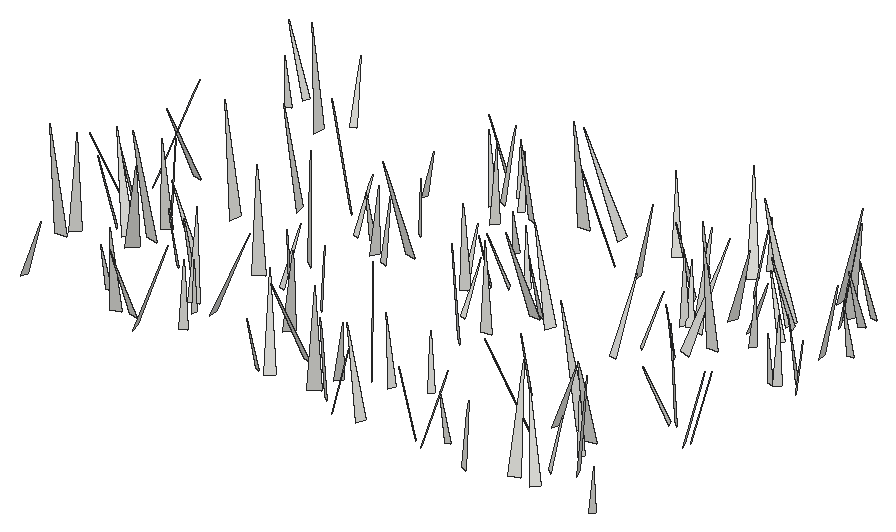
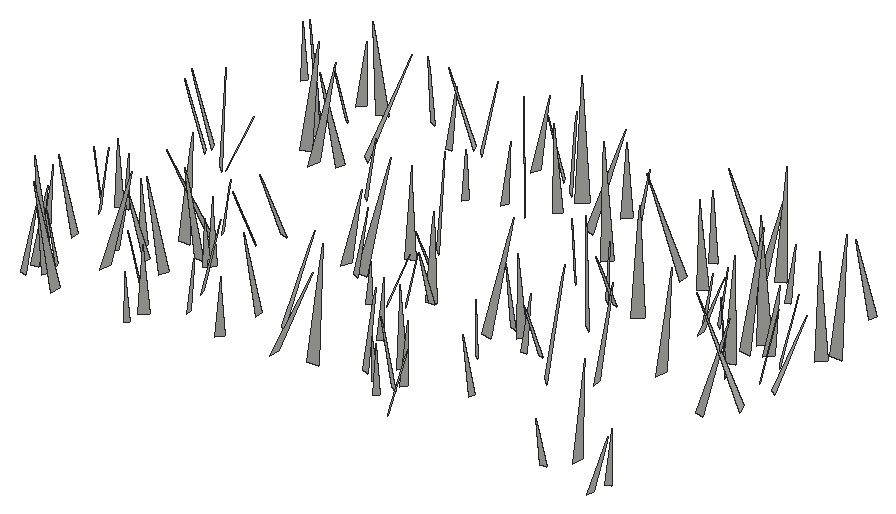
# SketchUp Ruby script. Lengths in inches.
U = 1.inch
M = Sketchup.active_model
def pt(a) = Geom::Point3d.new(a.map { |v| v * U })
def face(e, loops, mat)
  f = e.add_face(loops[0].map { |a| pt(a) })
  loops[1..].each { |l| e.add_face(l.map { |a| pt(a) }).erase! }
  f.material = f.back_material = mat if mat
  f
end
# faces: each face lists its corners as indices into pts; further lists are holes
def faces(e, pts, list, mat = nil) = list.each { |f| face(e, (f[0].is_a?(Array) ? f : [f]).map { |l| l.map { |i| pts[i] } }, mat) }
# xy, xz, yz: faces in a plane at the given z, y or x. An outline is a flat list of corners, or four numbers for a rectangle; further outlines are holes
def ring(l) = l.size == 4 ? [[l[0], l[1]], [l[2], l[1]], [l[2], l[3]], [l[0], l[3]]] : l.each_slice(2).to_a
def flat(e, list, mat, &to3) = list.each { |f| face(e, (f[0].is_a?(Array) ? f : [f]).map { |l| ring(l).map { |u, v| to3.(u, v) } }, mat) }
def xy(e, z, list, mat = nil) = flat(e, list, mat) { |x, y| [x, y, z] }
def xz(e, y, list, mat = nil) = flat(e, list, mat) { |x, z| [x, y, z] }
def yz(e, x, list, mat = nil) = flat(e, list, mat) { |y, z| [x, y, z] }
def lines(e, pts, list) = list.each { |a, b| e.add_line(pt(pts[a]), pt(pts[b])) }
# prism: a flat outline (further loops are holes) pulled along v
def prism(e, loops, v, mat = nil)
  f = face(e, loops, mat); d = Geom::Vector3d.new(v.map { |x| x * U })
  f.pushpull(f.normal.samedirection?(d) ? d.length : -d.length)
end
def box(e, o, s, mat = nil) = prism(e, [[o, [o[0] + s[0], o[1], o[2]], [o[0] + s[0], o[1] + s[1], o[2]], [o[0], o[1] + s[1], o[2]]]], [0, 0, s[2]], mat)
def at(x, y, z, deg = 0) = Geom::Transformation.translation(pt([x, y, z])) * Geom::Transformation.rotation(ORIGIN, Z_AXIS, deg.degrees)
def axes(o, x, y, z) = Geom::Transformation.new([*x, 0, *y, 0, *z, 0, *pt(o).to_a, 1])
def part(name) = M.definitions.add(name)
# library, detail: a bought-in or finely detailed component or shape, given as its bounding box
def library(name, o, s) = part(name).tap { |d| box(d.entities, o, s) }
def detail(e, o, s) = box(e.add_group.entities, o, s)
def put(e, d, t, mat = nil) = e.add_instance(d, t).tap { |i| i.material = mat if mat }
def group(e, t, mat = nil) = e.add_group.tap { |g| g.transformation = t; g.material = mat if mat }.entities
root = M.entities
c1 = part("fur_instance\#9")
p = [[0.8125,0,1.79],[0.67,-0.02,1.48],[0,-0.11,0],[0,0.11,0]]
faces(c1.entities,p,[[0,1,2,3]])
put(root,c1,axes([529.24,361.24,-21.66],[1.95895,3.98258,1.69888],[4.26762,-2.09086,-0.01944],[-0.73116,-1.53362,4.43825]))
put(root,c1,axes([548,362.49,-21.66],[2.54214,-2.62214,0.84113],[-2.70032,-2.59808,0.06187],[-0.53981,0.64801,3.65161]))
put(root,c1,axes([519.99,363.39,-21.66],[-3.55733,-3.55392,1.20149],[-3.66341,3.64755,-0.05732],[0.80828,0.89081,5.02808]))
put(root,c1,axes([508.05,362.3125,-21.66],[3.92442,2.27765,0.90763],[2.32456,-4.0011,-0.01041],[-0.77966,-0.46478,4.53747]))
put(root,c1,axes([512.18,362.6,-21.66],[-5.92125,2.00992,1.02968],[2.02644,6.00419,-0.06686],[0.99676,-0.26678,6.25272]))
put(root,c1,axes([521.57,362.67,-21.66],[5.13146,2.31605,0.71954],[2.33013,-5.17519,0.0403],[-0.67253,-0.25897,5.62978]))
put(root,c1,axes([472.16,365.39,-21.66],[3.11086,-6.46121,1.0779],[-6.53922,-3.13316,0.09147],[-0.38422,1.01124,7.17051]))
put(root,c1,axes([474.56,365.76,-21.66],[-0.49515,-5.81147,0.35136],[-5.82208,0.49376,-0.03799],[-0.0081,0.35331,5.8324]))
put(root,c1,axes([503,365.07,-21.66],[4.71718,-6.41333,2.08506],[-6.64537,-4.85367,0.10513],[-1.14777,1.74389,7.96063]))
put(root,c1,axes([505.4,364.37,-21.66],[-3.42106,-4.15596,2.05732],[-4.44833,3.66341,0.00339],[1.31032,1.58608,5.3829]))
put(root,c1,axes([523.79,364.9375,-21.66],[0.76269,-3.95415,0.89534],[-4.04548,-0.80213,-0.09639],[-0.26648,0.86018,4.02588]))
put(root,c1,axes([476.5625,363.62,-21.66],[6.39935,1.66924,0.57136],[1.67346,-6.42366,0.02366],[-0.55885,-0.12123,6.61343]))
put(root,c1,axes([494.44,364.85,-21.66],[-1.9321,-3.03286,0.9193],[-3.13143,1.99261,-0.00754],[0.48737,0.77951,3.596]))
put(root,c1,axes([538.63,363.23,-21.66],[-4.40287,4.25609,0.42122],[4.26988,4.40886,0.08361],[0.24458,-0.35298,6.12311]))
put(root,c1,axes([457.97,365.45,-21.66],[4.67852,-1.7119,0.20248],[-1.71617,-4.68064,0.08066],[-0.16239,0.14538,4.98123]))
put(root,c1,axes([535.25,363.49,-21.66],[-2.63415,6.93544,1.64719],[7.09873,2.71215,-0.06728],[0.64926,-1.51533,7.41852]))
put(root,c1,axes([496.4375,364.76,-21.66],[-4.20959,5.12778,0.85898],[5.1677,4.24809,-0.03415],[0.57165,-0.64206,6.63427]))
put(root,c1,axes([481.34,366.89,-21.66],[2.46407,-3.91283,1.91735],[-4.25122,-2.64198,0.07181],[-0.95581,1.66367,4.6235]))
put(root,c1,axes([503.83,368.89,-21.66],[4.00821,-3.73033,0.31245],[-3.73197,-4.01777,-0.09299],[-0.29215,0.14465,5.47471]))
put(root,c1,axes([497.75,370.3,-21.66],[-1.99035,-6.59495,0.1128],[-6.59501,1.99173,0.07994],[0.10913,0.08488,6.88828]))
put(root,c1,axes([537.77,367.13,-21.66],[1.92341,3.31368,0.82854],[3.39872,-1.95136,-0.08567],[-0.34002,-0.7604,3.83049]))
put(root,c1,axes([468.19,368.98,-21.66],[0.55845,-3.67703,0.59896],[-3.72525,-0.55803,0.04757],[-0.0423,0.59936,3.71889]))
put(root,c1,axes([540.7,368.91,-21.66],[5.91365,2.78735,2.33328],[2.94924,-6.28377,0.03183],[-2.12497,-0.96423,6.53755]))
put(root,c1,axes([530,373.12,-21.66],[-4.57477,-6.03245,0.25242],[-6.03633,4.57654,-0.02819],[0.13005,0.21817,7.57088]))
put(root,c1,axes([479.83,370.99,-21.66],[-3.27969,0.65416,1.38528],[0.68941,3.5533,-0.04576],[1.36808,-0.22237,3.34398]))
put(root,c1,axes([506.58,371.71,-21.66],[-5.8561,-4.67693,3.47291],[-5.12361,6.47844,0.0849],[2.77191,2.09401,7.49403]))
put(root,c1,axes([509.93,371.41,-21.66],[-4.33048,1.8912,1.2808],[1.94847,4.49129,-0.04381],[1.19187,-0.47097,4.72523]))
put(root,c1,axes([481.6875,372.3,-21.66],[7.09843,0.26187,0.16049],[0.26265,-7.10014,-0.03187],[-0.15921,-0.03777,7.10319]))
put(root,c1,axes([538.4,372.45,-21.66],[-3.29969,1.99263,1.18367],[2.06312,3.46364,-0.07948],[1.05601,-0.54058,3.85386]))
put(root,c1,axes([491.65,374.51,-21.66],[5.04429,-5.44094,0.7168],[-5.46997,-5.06343,0.05905],[-0.44381,0.56596,7.41924]))
put(root,c1,axes([478.23,372.85,-21.66],[-2.28357,5.70644,2.33564],[6.0895,2.47813,-0.10083],[0.96778,-2.12809,6.14557]))
put(root,c1,axes([514.42,373.48,-21.66],[-2.6188,2.85202,1.01974],[2.95253,2.70449,0.01846],[0.67563,-0.76402,3.87193]))
put(root,c1,axes([537.0625,375.97,-21.66],[1.68994,-6.65431,0.98946],[-6.7239,-1.70391,0.02495],[-0.21912,0.96522,6.8655]))
put(root,c1,axes([455.31,375.85,-21.66],[-0.06707,-7.91469,2.47451],[-8.29222,0.04381,-0.08466],[-0.06773,2.47503,7.91452]))
put(root,c1,axes([531.44,376.33,-21.66],[5.62437,-1.82953,0.08499],[-1.8284,-5.62476,-0.0835],[-0.10665,-0.05312,5.91386]))
put(root,c1,axes([463.97,378.83,-21.66],[5.44226,-5.9088,0.26751],[-5.91243,-5.44486,0.01623],[-0.16928,0.20777,8.03317]))
put(root,c1,axes([456.17,377.63,-21.66],[-4.86484,4.13925,3.64162],[4.78109,5.5858,0.03796],[2.74517,-2.39309,6.38738]))
put(root,c1,axes([471.11,378.6,-21.66],[-2.39364,-3.13142,1.17859],[-3.27618,2.48779,-0.04385],[0.67935,0.9641,3.94124]))
put(root,c1,axes([534.29,377.95,-21.66],[-8.05212,1.79962,1.36323],[1.82873,8.16018,0.02927],[1.32393,-0.32629,8.25072]))
put(root,c1,axes([473.27,378.75,-21.66],[-3.37227,-0.8607,0.92289],[-0.91034,3.4828,-0.07828],[0.87397,0.30665,3.4795]))
put(root,c1,axes([464.56,381.79,-21.66],[-1.19832,-8.06423,2.00487],[-8.30399,1.23724,0.01324],[0.30817,1.98109,8.15276]))
put(root,c1,axes([524,380.75,-21.66],[-2.56443,-3.19615,1.19823],[-3.34404,2.653,-0.08027],[0.6845,0.98675,4.09698]))
put(root,c1,axes([459.35,381.61,-21.66],[-3.89073,-3.2521,0.98713],[-3.3181,3.95947,-0.03367],[0.73538,0.65937,5.07078]))
put(root,c1,axes([491.41,380.99,-21.66],[3.14318,2.78213,1.66083],[2.96777,-3.40061,0.07991],[-1.30037,-1.03624,4.19683]))
put(root,c1,axes([471.76,381.4,-21.66],[-5.15429,0.32159,0.0951],[0.32057,5.15491,-0.05731],[0.09848,0.05128,5.164]))
put(root,c1,axes([461.82,380.58,-21.66],[-5.31881,4.24046,0.31909],[4.24772,5.322,0.07866],[0.20039,-0.26047,6.80184]))
put(root,c1,axes([485.46,382.375,-21.66],[-2.49049,-3.07283,1.62396],[-3.33154,2.67981,-0.03854],[0.99012,1.28779,3.95516]))
put(root,c1,axes([480.12,383.01,-21.66],[4.03772,-5.94106,3.0996],[-6.44975,-4.42725,-0.08397],[-1.8178,2.512,7.18278]))
put(root,c1,axes([546.38,382.27,-21.66],[4.95919,2.18923,1.00137],[2.21006,-5.04934,0.09393],[-0.95452,-0.31696,5.4201]))
put(root,c1,axes([484.25,382.3,-21.66],[1.13394,4.06883,0.24777],[4.07369,-1.14042,0.08414],[-0.14769,-0.216,4.22305]))
put(root,c1,axes([464.42,384.96,-21.66],[2.81734,-6.20209,1.85033],[-6.41792,-2.93797,-0.07572],[-0.83667,1.65211,6.81158]))
put(root,c1,axes([546.32,383.74,-21.66],[4.35259,2.65064,0.87547],[2.69973,-4.40951,-0.0717],[-0.70982,-0.51745,5.09567]))
put(root,c1,axes([541.75,385.39,-21.66],[-3.79405,-1.81524,0.00607],[-1.81515,3.79397,0.03081],[0.01877,-0.02517,4.20582]))
put(root,c1,axes([509.16,385.39,-21.66],[3.99412,4.65299,3.2629],[5.30006,-4.48907,-0.08624],[-2.05092,-2.53923,6.13155]))
put(root,c1,axes([458.83,385.99,-21.66],[-4.42725,-2.60663,1.07476],[-2.66002,4.52485,0.01676],[0.93485,0.53053,5.13759]))
put(root,c1,axes([455.86,387.26,-21.66],[-3.26059,-4.43586,0.10579],[-4.43536,3.26207,0.0775],[0.12511,0.03932,5.50476]))
put(root,c1,axes([542.23,385.87,-21.66],[-4.17203,-5.0841,2.64194],[-5.48144,4.49304,-0.00972],[1.66784,2.04897,6.57676]))
put(root,c1,axes([462.82,387.72,-21.66],[4.34542,2.75412,2.00138],[2.98226,-4.64462,-0.0836],[-1.6422,-1.14703,5.14401]))
put(root,c1,axes([510.52,389.04,-21.66],[-1.61639,5.70202,2.80279],[6.31476,1.76115,0.05886],[0.70173,-2.71416,5.92641]))
put(root,c1,axes([483.26,388.88,-21.66],[4.5767,5.68819,3.18986],[6.17982,-5.02762,0.09872],[-2.08339,-2.41752,7.30013]))
put(root,c1,axes([505.85,390.25,-21.66],[0.74131,3.87524,0.12897],[3.87698,-0.74271,0.03187],[-0.05555,-0.12068,3.94537]))
put(root,c1,axes([469.18,392.15,-21.66],[-7.46216,1.5868,2.36089],[1.65538,7.81249,-0.01867],[2.31332,-0.47194,7.62898]))
put(root,c1,axes([512.72,395.6,-21.66],[-0.43608,-7.58063,0.50958],[-7.59761,0.43802,0.01424],[0.04352,0.50791,7.59315]))
put(root,c1,axes([456.28,392.71,-21.66],[7.55875,3.30018,0.58934],[3.3113,-7.57673,-0.04195],[-0.52327,-0.27436,8.24768]))
put(root,c1,axes([459.4,397.1,-21.66],[-1.29873,-6.18935,0.13887],[-6.18983,1.30082,0.08883],[0.11547,0.11765,6.32352]))
put(root,c1,axes([487.88,395.7,-21.66],[4.42383,-2.92058,1.2942],[-2.99041,-4.56361,-0.07677],[-1.12348,0.64702,5.30039]))
put(root,c1,axes([490.07,394.59,-21.66],[-1.46329,-3.87448,2.4887],[-4.52721,1.6881,-0.03379],[0.84239,2.34204,4.14146]))
put(root,c1,axes([501.87,395.7,-21.66],[2.29625,-5.32789,2.30917],[-5.72704,-2.48806,-0.04565],[-0.95905,2.10109,5.80148]))
put(root,c1,axes([513.0625,396.25,-21.66],[-1.72033,-4.15588,1.09836],[-4.2769,1.77348,0.01157],[0.4311,1.01028,4.49785]))
put(root,c1,axes([515.79,394.77,-21.66],[-6.07575,2.79462,0.62219],[2.80321,6.10345,-0.04049],[0.58225,-0.22305,6.68752]))
put(root,c1,axes([491.56,397.99,-21.66],[-1.16201,-7.65185,1.0654],[-7.72512,1.16361,-0.06847],[0.09162,1.06366,7.73928]))
put(root,c1,axes([526.125,393.89,-21.66],[0.97806,5.36378,0.25201],[5.36787,-0.98334,0.09641],[-0.14015,-0.23057,5.45137]))
put(root,c1,axes([501.68,395.87,-21.66],[0.3484,4.1984,0.59349],[4.23915,-0.35779,0.04247],[-0.09183,-0.58788,4.21262]))
put(root,c1,axes([485.5,398.38,-21.66],[0.8315,-3.67241,0.7269],[-3.73531,-0.86356,-0.09004],[-0.24991,0.6885,3.76429]))
put(root,c1,axes([503.7,398.29,-21.66],[2.36967,1.89121,2.13493],[2.35412,-2.86396,-0.07595],[-1.61018,-1.40392,3.03088]))
put(root,c1,axes([532.14,398.15,-21.66],[-3.28529,-1.60429,1.12724],[-1.66632,3.44368,0.04462],[1.03333,0.45264,3.6558]))
put(root,c1,axes([473.92,398.69,-21.66],[-6.8866,-1.44069,2.04712],[-1.4724,7.17733,0.09795],[2.02444,0.3193,7.035]))
put(root,c1,axes([505.68,399.42,-21.66],[-3.47734,-1.80435,0.22841],[-1.8088,3.48242,-0.02761],[0.19,0.12974,3.9175]))
put(root,c1,axes([527.41,397.76,-21.66],[2.54826,3.20038,0.28055],[3.20908,-2.5526,-0.02947],[-0.15164,-0.23787,4.09087]))
put(root,c1,axes([483.3,397.81,-21.66],[0.89706,4.01856,0.51185],[4.05094,-0.89322,-0.08685],[-0.02607,-0.51851,4.11655]))
put(root,c1,axes([545.09,400.62,-21.66],[-0.48209,-3.49328,1.24378],[-3.69826,0.54426,0.09516],[0.26993,1.21786,3.5251]))
put(root,c1,axes([546.02,400.77,-21.66],[-2.69115,3.5868,1.84623],[3.86426,2.92918,-0.05799],[1.15809,-1.43902,4.48375]))
put(root,c1,axes([548.86,400.77,-21.66],[-2.22453,-2.28888,1.93607],[-2.6411,2.63697,0.08289],[1.41842,1.32035,3.19071]))
put(root,c1,axes([479,402.16,-21.66],[-5.20637,-5.83633,2.28098],[-6.06397,5.44004,0.07832],[1.57922,1.64775,7.82067]))
put(root,c1,axes([507.56,400.64,-21.66],[-2.46678,3.0111,0.36551],[3.02886,2.4705,0.08915],[0.1623,-0.33942,3.8915]))
put(root,c1,axes([534.27,402.83,-21.66],[0.04247,-7.07988,2.41623],[-7.48051,-0.06275,-0.05238],[-0.06984,2.41579,7.07981]))
put(root,c1,axes([489.21,402.79,-21.66],[-2.0645,-2.99831,1.70133],[-3.28642,2.31061,0.08412],[1.04107,1.34824,3.63936]))
put(root,c1,axes([547.11,403.16,-21.66],[-3.81411,-2.18756,1.38745],[-2.30966,3.98998,-0.05835],[1.17299,0.74331,4.39652]))
put(root,c1,axes([532.3125,400.04,-21.66],[2.76635,7.35948,0.05567],[7.35952,-2.76581,-0.07342],[0.04914,-0.07794,7.86188]))
put(root,c1,axes([500.875,406.72,-21.66],[2.15592,-3.18911,0.31319],[-3.19535,-2.16794,-0.07942],[-0.24138,0.21478,3.84865]))
put(root,c1,axes([528.03,405.37,-21.66],[-3.99726,2.72851,1.81883],[2.89094,4.28575,-0.07581],[1.5477,-0.9584,4.83912]))
put(root,c1,axes([537.71,406.39,-21.66],[-2.80028,2.24736,2.49663],[2.73085,3.4158,-0.01176],[1.95607,-1.55147,3.59055]))
put(root,c1,axes([530.31,404.91,-21.66],[0.3651,6.79595,1.75212],[7.01816,-0.34958,-0.10649],[0.01583,-1.75528,6.80491]))
put(root,c1,axes([528.58,405.61,-21.66],[-2.41477,3.3901,0.55663],[3.41153,2.44646,-0.10002],[0.40504,-0.3947,4.161]))
put(root,c1,axes([535.15,409.04,-21.66],[4.26673,-0.51352,0.23406],[-0.5171,-4.27238,0.05285],[-0.22604,0.08052,4.29719]))
put(root,c1,axes([531.66,410.14,-21.66],[5.79925,-1.98106,0.58125],[-1.98372,-5.82701,-0.06806],[-0.57211,0.1232,6.12791]))
put(root,c1,axes([545.76,409.65,-21.66],[5.31059,0.52385,1.16283],[0.52648,-5.43598,0.04446],[-1.16164,-0.06886,5.33618]))
put(root,c1,axes([483.73,410.54,-21.66],[3.66443,-1.25509,0.51627],[-1.25966,-3.69872,-0.05095],[-0.50503,0.11865,3.87307]))
put(root,c1,axes([539.72,409.38,-21.66],[-3.84574,2.31871,0.01808],[2.31862,3.84577,-0.02193],[0.02681,0.00945,4.49062]))
put(root,c1,axes([494.51,410.63,-21.66],[4.30224,-3.16543,2.15858],[-3.43037,-4.62804,0.05027],[-1.70646,1.32286,5.34104]))
put(root,c1,axes([511.87,411.94,-21.66],[-4.79453,-5.10071,1.01007],[-5.15614,4.84133,-0.02673],[0.67211,0.75447,7.00029]))
put(root,c1,axes([524.97,410.99,-21.66],[-4.98874,-1.77944,1.14235],[-1.81158,5.1064,0.04294],[1.09068,0.3424,5.29642]))
put(root,c1,axes([548.35,411.91,-21.66],[1.07632,-4.38935,0.89904],[-4.4763,-1.09335,0.02097],[-0.19334,0.87825,4.51934]))
put(root,c1,axes([516.25,411.05,-21.66],[5.41159,0.09186,1.28906],[0.07062,-5.56242,0.09991],[-1.29039,0.08081,5.41145]))
put(root,c1,axes([538.75,412.99,-21.66],[-4.66141,-1.64687,0.68606],[-1.65466,4.70851,0.06011],[0.66704,0.1713,4.94341]))
put(root,c1,axes([497.46,413.98,-21.66],[-1.75963,-5.21212,1.71135],[-5.46295,1.82898,-0.04671],[0.50104,1.63703,5.50093]))
put(root,c1,axes([537.97,413.45,-21.66],[-8.02945,1.44749,0.94959],[1.4539,8.08421,-0.0293],[0.93976,-0.13944,8.15883]))
put(root,c1,axes([491.58,413.88,-21.66],[-4.02288,2.74208,1.38872],[2.85785,4.17888,0.02734],[1.13147,-0.80565,4.86845]))
put(root,c1,axes([463.69,415.2,-21.66],[-6.94561,0.7265,2.56424],[0.79665,7.39636,0.06233],[2.54332,-0.33278,6.98322]))
put(root,c1,axes([503.6,416.42,-21.66],[1.30407,-7.61557,2.3618],[-7.95747,-1.39423,-0.10194],[-0.50366,2.30972,7.72574]))
put(root,c1,axes([495.13,414.96,-21.66],[-1.61358,3.38665,0.61033],[3.4322,1.63258,0.01498],[0.24881,-0.55751,3.75138]))
put(root,c1,axes([523.21,415.83,-21.66],[-3.75742,-0.36081,1.22113],[-0.40687,3.94545,-0.08619],[1.20657,0.20686,3.77372]))
put(root,c1,axes([492.12,415.17,-21.66],[2.52877,4.50107,1.40807],[4.66336,-2.62485,0.01569],[-0.70386,-1.21962,5.16276]))
put(root,c1,axes([544.91,418.4375,-21.66],[1.17594,-4.92519,0.34785],[-4.93492,-1.18388,-0.07952],[-0.1583,0.31979,5.06301]))
put(root,c1,axes([542.87,416.7,-21.66],[3.30994,1.56111,0.94089],[1.62723,-3.40964,-0.0672],[-0.82125,-0.46405,3.659]))
put(root,c1,axes([529.89,416.34,-21.66],[3.54809,3.00738,1.07129],[3.07779,-3.64774,0.04651],[-0.84804,-0.65624,4.65093]))
put(root,c1,axes([457.1,417.47,-21.66],[1.04159,-3.44564,1.2731],[-3.64709,-1.12789,-0.06873],[-0.4381,1.19732,3.59897]))
put(root,c1,axes([508.86,417.24,-21.66],[-7.40149,0.22253,0.007],[0.22253,7.40149,0.00759],[0.00677,-0.0078,7.40483]))
put(root,c1,axes([492.89,417.63,-21.66],[1.88047,-2.78184,1.95652],[-3.20631,-2.19563,-0.04014],[-1.13412,1.59479,3.35756]))
put(root,c1,axes([542.47,418.95,-21.66],[7.05562,-2.47543,1.6862],[-2.53392,-7.23407,-0.01726],[-1.59697,0.54154,7.47725]))
put(root,c1,axes([516.67,418.05,-21.66],[-3.66348,3.88372,0.60062],[3.90017,3.69385,-0.09601],[0.48235,-0.37054,5.33808]))
put(root,c1,axes([488.92,420.18,-21.66],[-3.66395,-2.75565,0.79106],[-2.79858,3.7164,-0.01609],[0.62239,0.48852,4.58453]))
put(root,c1,axes([544.86,420.78,-21.66],[-0.84306,-4.44176,0.86686],[-4.52258,0.85891,0.00263],[0.16427,0.85115,4.52106]))
put(root,c1,axes([466.31,418.57,-21.66],[-1.50833,4.20798,0.27956],[4.21722,1.50618,0.08227],[0.01672,-0.29093,4.46939]))
put(root,c1,axes([457.63,420.3,-21.66],[-4.98087,1.16288,0.32288],[1.15979,4.99131,-0.08543],[0.33384,0.00996,5.1141]))
put(root,c1,axes([527.28,419.46,-21.66],[-4.42637,5.44798,0.10976],[5.44745,4.42761,-0.08267],[0.13338,-0.03304,7.019]))
put(root,c1,axes([539.19,421.65,-21.66],[7.16515,0.1083,1.44204],[0.09788,-7.3087,0.06254],[-1.44279,0.042,7.1657]))
put(root,c1,axes([527.66,422.27,-21.66],[1.56835,-2.82264,1.69633],[-3.20586,-1.73838,0.07137],[-0.75322,1.52161,3.2283]))
